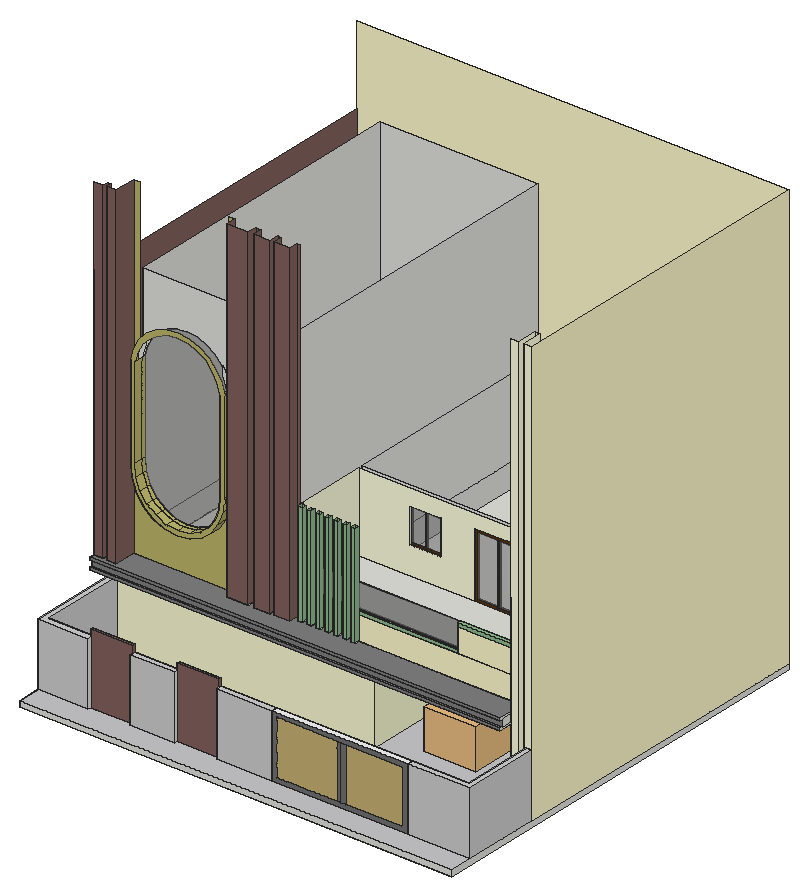
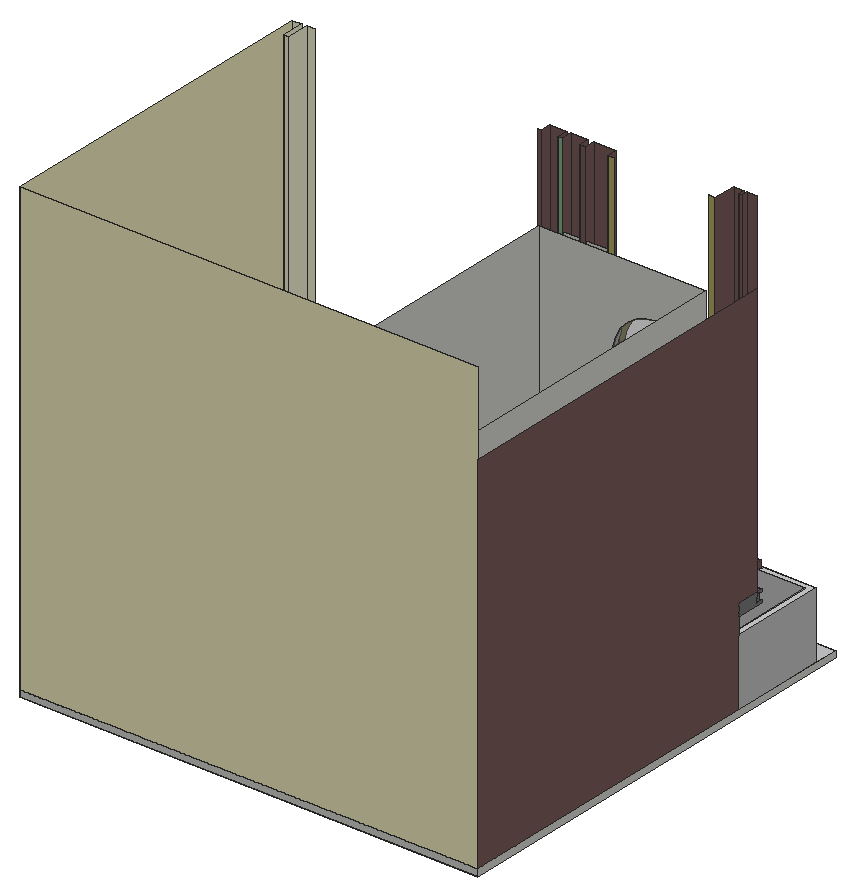
# SketchUp Ruby script. Lengths in inches.
U = 1.inch
M = Sketchup.active_model
def pt(a) = Geom::Point3d.new(a.map { |v| v * U })
def face(e, loops, mat)
  f = e.add_face(loops[0].map { |a| pt(a) })
  loops[1..].each { |l| e.add_face(l.map { |a| pt(a) }).erase! }
  f.material = f.back_material = mat if mat
  f
end
# faces: each face lists its corners as indices into pts; further lists are holes
def faces(e, pts, list, mat = nil) = list.each { |f| face(e, (f[0].is_a?(Array) ? f : [f]).map { |l| l.map { |i| pts[i] } }, mat) }
# xy, xz, yz: faces in a plane at the given z, y or x. An outline is a flat list of corners, or four numbers for a rectangle; further outlines are holes
def ring(l) = l.size == 4 ? [[l[0], l[1]], [l[2], l[1]], [l[2], l[3]], [l[0], l[3]]] : l.each_slice(2).to_a
def flat(e, list, mat, &to3) = list.each { |f| face(e, (f[0].is_a?(Array) ? f : [f]).map { |l| ring(l).map { |u, v| to3.(u, v) } }, mat) }
def xy(e, z, list, mat = nil) = flat(e, list, mat) { |x, y| [x, y, z] }
def xz(e, y, list, mat = nil) = flat(e, list, mat) { |x, z| [x, y, z] }
def yz(e, x, list, mat = nil) = flat(e, list, mat) { |y, z| [x, y, z] }
def lines(e, pts, list) = list.each { |a, b| e.add_line(pt(pts[a]), pt(pts[b])) }
# prism: a flat outline (further loops are holes) pulled along v
def prism(e, loops, v, mat = nil)
  f = face(e, loops, mat); d = Geom::Vector3d.new(v.map { |x| x * U })
  f.pushpull(f.normal.samedirection?(d) ? d.length : -d.length)
end
def box(e, o, s, mat = nil) = prism(e, [[o, [o[0] + s[0], o[1], o[2]], [o[0] + s[0], o[1] + s[1], o[2]], [o[0], o[1] + s[1], o[2]]]], [0, 0, s[2]], mat)
def at(x, y, z, deg = 0) = Geom::Transformation.translation(pt([x, y, z])) * Geom::Transformation.rotation(ORIGIN, Z_AXIS, deg.degrees)
def axes(o, x, y, z) = Geom::Transformation.new([*x, 0, *y, 0, *z, 0, *pt(o).to_a, 1])
def part(name) = M.definitions.add(name)
# library, detail: a bought-in or finely detailed component or shape, given as its bounding box
def library(name, o, s) = part(name).tap { |d| box(d.entities, o, s) }
def detail(e, o, s) = box(e.add_group.entities, o, s)
def put(e, d, t, mat = nil) = e.add_instance(d, t).tap { |i| i.material = mat if mat }
def group(e, t, mat = nil) = e.add_group.tap { |g| g.transformation = t; g.material = mat if mat }.entities
root = M.entities
M.materials.add("[0043_SaddleBrown]").color = [130, 97, 94]
M.materials.add("[0050_LemonChiffon]").color = [255, 250, 205]
M.materials.add("[0054_LightYellow]").color = [255, 255, 224]
M.materials.add("[0055_LightGoldenrodYellow]").color = [250, 250, 210]
M.materials.add("[0057_DarkKhaki]").color = [189, 183, 107]
M.materials.add("[0072_DarkSeaGreen]").color = [143, 188, 143]
M.materials.add("[0086_MediumAquamarine]").color = [102, 205, 170]
M.materials.add("[0118_Thistle]").color = [216, 191, 216]
M.materials.add("[0129_WhiteSmoke]").color = [245, 245, 245]
M.materials.add("[0133_Gray]").color = [128, 128, 128]
M.materials.add("[Cladding Siding White]").color = [207, 207, 207]
M.materials.add("[Color C08]").color = [102, 51, 0]
M.materials.add("[Color M05]").color = [114, 114, 114]
M.materials.add("[Metal Seamed]").color = [118, 119, 115]
M.materials.add("[Polished Concrete New]").color = [200, 200, 203]
M.materials.add("[Translucent Glass Gray]").color = [128, 128, 128]
M.materials["[Translucent Glass Gray]"].alpha = 0.5
M.materials.add("[Window Covering 02]").color = [199, 178, 115]
c1 = library("custom el camino",[47.5625,9.86,-8],[222.64,79.59,60.9375])
c2 = part("Group\#1")
xy(c2.entities,0,[[0,0,81.875,4.3125]],"[Color C08]")
xy(c2.entities,4.13,[[4.13,0,38.5,0.0625],[38.5,0,42.19,0.0625],[42.19,0,77.74,0.0625],[4.13,0.0625,38.5,4.3125],[38.5,0.0625,42.19,4.3125],
  [42.19,0.0625,77.74,4.3125]],"[Color C08]")
xy(c2.entities,128.34,[[4.13,0,38.5,0.0625],[42.19,0,77.74,0.0625],[4.13,0.0625,38.5,4.3125],[42.19,0.0625,77.74,4.3125]],"[Color C08]")
xy(c2.entities,132.48,[[0,0,81.875,4.3125]],"[Color C08]")
xz(c2.entities,0,[[[0,0,81.875,132.48],[4.13,4.13,4.13,128.34,38.5,128.34,38.5,4.13,42.19,4.13,42.19,128.34,77.74,128.34,77.74,4.13]]],"[Color C08]")
xz(c2.entities,0.0625,[[4.13,4.13,38.5,128.34],[42.19,4.13,77.74,128.34]],"[Translucent Glass Gray]")
xz(c2.entities,4.3125,[[[0,0,81.875,132.48],[4.13,4.13,77.74,4.13,77.74,128.34,42.19,128.34,42.19,4.13,38.5,4.13,38.5,128.34,4.13,128.34]]],"[Color C08]")
yz(c2.entities,0,[[0,0,4.3125,132.48]],"[Color C08]")
yz(c2.entities,4.13,[[0,4.13,0.0625,128.34],[0.0625,4.13,4.3125,128.34]],"[Color C08]")
yz(c2.entities,38.5,[[0,4.13,0.0625,128.34],[0.0625,4.13,4.3125,128.34]],"[Color C08]")
yz(c2.entities,42.19,[[0,4.13,0.0625,128.34],[0.0625,4.13,4.3125,128.34]],"[Color C08]")
yz(c2.entities,77.74,[[0,4.13,0.0625,128.34],[0.0625,4.13,4.3125,128.34]],"[Color C08]")
yz(c2.entities,81.875,[[0,0,4.3125,132.48]],"[Color C08]")
xy(root,0,[[0,0,657.3125,34.75],[0,34.75,657.3125,640.8125]])
xy(root,9,[[0,34.75,0,173.6875,9,173.6875,9,43.75,356.0625,43.75,356.0625,34.75,271.24,34.75,271.24,39.125,207.56,39.125,207.56,34.75,139.74,34.75,139.74,39.125,76.06,39.125,76.06,34.75],[562.44,35.125,562.44,43.75,648.3125,43.75,648.3125,152.625,657.3125,152.625,657.3125,35.125],[[624.625,152.625,624.625,631.8125,401.125,631.8125,401.125,173.6875,0,173.6875,0,640.8125,657.3125,640.8125,657.3125,152.625,644.16,152.625,644.16,183.8125,637.14,183.8125,637.14,152.625],[42.625,179.6875,395.125,631.8125]],[42.625,179.6875,395.125,631.8125]])
xy(root,9,[[0,0,657.3125,0,657.3125,35.125,562.44,35.125,562.44,34.75,271.24,34.75,271.24,39.125,207.56,39.125,207.56,34.75,139.74,34.75,139.74,39.125,76.06,39.125,76.06,34.75,0,34.75],[356.0625,34.75,562.44,43.75],[9,43.75,648.3125,43.75,648.3125,152.625,644.16,152.625,644.16,183.8125,637.14,183.8125,637.14,152.625,624.625,152.625,624.625,631.8125,401.125,631.8125,401.125,173.6875,9,173.6875]],"[Polished Concrete New]")
xy(root,105,[[356.0625,34.75,562.44,43.75]],"[0129_WhiteSmoke]")
xy(root,105,[[0,34.75,76.06,34.75,76.06,43.75,9,43.75,9,173.6875,0,173.6875],[139.74,34.75,207.56,43.75],[271.24,34.75,356.0625,43.75],[562.44,35.125,657.3125,35.125,657.3125,152.625,648.3125,152.625,648.3125,43.75,562.44,43.75]],"[Cladding Siding White]")
xy(root,115.875,[[76.06,39.125,139.74,43.75],[207.56,39.125,271.24,43.75]],"[0043_SaddleBrown]")
xy(root,123,[[42.625,179.6875,395.125,631.8125]])
xy(root,129,[[401.125,132.75,624.625,631.8125],[42.625,179.6875,395.125,631.8125]])
xy(root,129,[[0,132.75,401.125,173.6875]],"[0133_Gray]")
xy(root,132.4375,[[0,137,0,140.625,14.17,140.625,14.17,148.6875,19.125,148.6875,19.125,140.625,33.625,140.625,33.625,173.6875,187.68,173.6875,187.68,159.3125,219.81,159.3125,219.81,173.6875,228.25,173.6875,228.25,159.3125,252.93,159.3125,252.93,173.6875,289.55,173.6875,289.55,167.4375,295.8,167.4375,295.8,173.6875,302.98,173.6875,302.98,167.4375,309.23,167.4375,309.23,173.6875,316.42,173.6875,316.42,167.4375,322.67,167.4375,322.67,173.6875,329.86,173.6875,329.86,167.4375,336.11,167.4375,336.11,173.6875,343.3,173.6875,343.3,167.4375,349.55,167.4375,349.55,173.6875,356.73,173.6875,356.73,167.4375,362.98,167.4375,362.98,173.6875,370.17,173.6875,370.17,167.4375,376.42,167.4375,376.42,173.6875,624.625,173.6875,624.625,137]])
xy(root,132.4375,[[0,132.75,624.625,137]],"[0133_Gray]")
xy(root,142.6875,[[0,137,0,140.625,14.17,140.625,14.17,148.6875,19.125,148.6875,19.125,140.625,33.625,140.625,33.625,173.6875,187.68,173.6875,187.68,159.3125,219.81,159.3125,219.81,173.6875,228.25,173.6875,228.25,159.3125,252.93,159.3125,252.93,173.6875,289.55,173.6875,289.55,167.4375,295.8,167.4375,295.8,173.6875,302.98,173.6875,302.98,167.4375,309.23,167.4375,309.23,173.6875,316.42,173.6875,316.42,167.4375,322.67,167.4375,322.67,173.6875,329.86,173.6875,329.86,167.4375,336.11,167.4375,336.11,173.6875,343.3,173.6875,343.3,167.4375,349.55,167.4375,349.55,173.6875,356.73,173.6875,356.73,167.4375,362.98,167.4375,362.98,173.6875,370.17,173.6875,370.17,167.4375,376.42,167.4375,376.42,173.6875,624.625,173.6875,624.625,137]])
xy(root,142.6875,[[0,132.75,624.625,137]],"[0133_Gray]")
xy(root,146,[[0,140.625,14.17,140.625,14.17,148.6875,19.125,148.6875,19.125,140.625,33.625,140.625,33.625,173.6875,0,173.6875],[289.55,167.4375,295.8,173.6875],[302.98,167.4375,309.23,173.6875],[316.42,167.4375,322.67,173.6875],[329.86,167.4375,336.11,173.6875],
  [343.3,167.4375,349.55,173.6875],[356.73,167.4375,362.98,173.6875],[370.17,167.4375,376.42,173.6875],[42.625,179.6875,282.1875,631.8125],[287.625,291.75,624.625,631.8125]])
xy(root,146,[[0,132.75,624.625,132.75,624.625,173.6875,376.42,173.6875,376.42,167.4375,370.17,167.4375,370.17,173.6875,362.98,173.6875,362.98,167.4375,356.73,167.4375,356.73,173.6875,349.55,173.6875,349.55,167.4375,343.3,167.4375,343.3,173.6875,336.11,173.6875,336.11,167.4375,329.86,167.4375,329.86,173.6875,322.67,173.6875,322.67,167.4375,316.42,167.4375,316.42,173.6875,309.23,173.6875,309.23,167.4375,302.98,167.4375,302.98,173.6875,295.8,173.6875,295.8,167.4375,289.55,167.4375,289.55,173.6875,252.93,173.6875,252.93,159.3125,228.25,159.3125,228.25,173.6875,219.81,173.6875,219.81,159.3125,187.68,159.3125,187.68,173.6875,33.625,173.6875,33.625,140.625,19.125,140.625,19.125,148.6875,14.17,148.6875,14.17,140.625,0,140.625]],"[0133_Gray]")
xy(root,146.3125,[[258.81,159.3125,282.62,173.6875]])
xy(root,182,[[287.625,173.6875,526.86,179.6875],[526.86,173.6875,624.625,179.6875],[287.625,179.6875,624.625,179.6875,624.625,285.75,536.61,285.75,536.61,291.75,463.98,291.75,463.98,285.75,287.625,285.75]])
xy(root,187.125,[[287.625,177.42,526.86,178.24],[287.625,178.24,526.86,179.6875]])
xy(root,187.125,[[287.625,173.6875,526.86,177.42]],"[0072_DarkSeaGreen]")
xy(root,218,[[526.86,173.6875,624.625,179.6875]])
xy(root,224.1875,[[526.86,173.6875,624.625,179.6875]],"[0072_DarkSeaGreen]")
xy(root,224.1875,[[287.625,177.42,526.86,178.24]],"[Metal Seamed]")
xy(root,224.4,[[364.57,285.75,412.01,291.75]])
xy(root,224.5625,[[287.625,177.42,526.86,178.24]],"[Metal Seamed]")
xy(root,276.72,[[364.57,285.75,412.01,291.75]])
xy(root,280.8125,[[463.98,285.75,536.61,291.75]])
xz(root,0,[[0,0,657.3125,9]])
xz(root,34.75,[[0,9,76.06,105],[139.74,9,207.56,105],[271.24,9,356.0625,105]],"[Cladding Siding White]")
xz(root,34.75,[[[356.0625,9,562.44,105],[362.9,15.84,555.61,98.16]],[454.57,15.84,461.28,98.16],[461.28,15.84,467.98,98.16]],"[Color M05]")
xz(root,34.75,[[362.9,15.84,454.57,98.16],[467.98,15.84,555.61,98.16]],"[Window Covering 02]")
xz(root,35.125,[[562.44,9,657.3125,105]],"[Cladding Siding White]")
xz(root,39.125,[[76.06,9,139.74,115.875],[207.56,9,271.24,115.875]],"[0043_SaddleBrown]")
xz(root,43.75,[[76.06,105,139.74,115.875],[207.56,105,271.24,115.875]],"[0043_SaddleBrown]")
xz(root,43.75,[[356.0625,9,562.44,105]],"[0129_WhiteSmoke]")
xz(root,43.75,[[9,9,356.0625,105],[562.44,9,648.3125,105]],"[Cladding Siding White]")
xz(root,132.75,[[0,129,624.625,132.4375],[0,142.6875,624.625,146]],"[0133_Gray]")
xz(root,137,[[0,132.4375,624.625,142.6875]],"[0133_Gray]")
xz(root,140.625,[[0,132.4375,14.17,142.6875],[19.125,132.4375,33.625,142.6875],[0,142.6875,14.17,146],[19.125,142.6875,33.625,146]])
xz(root,140.625,[[0,146,14.17,655],[19.125,146,33.625,655]],"[0043_SaddleBrown]")
xz(root,148.6875,[[14.17,132.4375,19.125,142.6875],[14.17,142.6875,19.125,146]])
xz(root,148.6875,[[14.17,146,19.125,655]],"[0043_SaddleBrown]")
xz(root,152.625,[[648.3125,9,657.3125,105]])
xz(root,152.625,[[624.625,9,637.14,655],[644.16,9,648.3125,9,648.3125,105,657.3125,105,657.3125,655,644.16,655]],"[0054_LightYellow]")
xz(root,159.3125,[[187.68,132.4375,219.81,142.6875],[228.25,132.4375,252.93,142.6875],[187.68,142.6875,219.81,146],[228.25,142.6875,252.93,146]])
xz(root,159.3125,[[187.68,146,219.81,655],[228.25,146,252.93,655],[258.81,146.3125,282.62,655]],"[0043_SaddleBrown]")
xz(root,160.875,[[[111.04,201.47,130.34,204.13,148.21,211.9,163.32,224.21,174.54,240.15,181.03,258.52,182.32,277.97,182.32,417.32,177.88,433.82,169.67,448.8125,158.17,461.45,144.02,471.02,128,476.98,111.04,479.01,94.07,476.98,78.06,471.02,63.9,461.45,52.4,448.8125,44.2,433.82,39.76,417.32,39.76,277.97,41.05,258.52,47.54,240.15,58.76,224.21,73.86,211.9,91.73,204.13],[111.04,208.61,93.66,211,77.58,218,63.98,229.08,53.88,243.43,48.04,259.96,46.83,278.2,46.83,416.39,50.81,431.17,58.2,444.68,68.5625,456.0625,81.32,464.6875,95.75,470.0625,111.04,471.89,126.33,470.0625,140.75,464.6875,153.51,456.0625,163.875,444.68,171.27,431.17,175.25,416.39,175.25,278.2,174.04,259.96,168.19,243.43,158.1,229.08,144.5,218,128.41,211]]],"[0057_DarkKhaki]")
xz(root,167.4375,[[289.55,132.4375,295.8,142.6875],[302.98,132.4375,309.23,142.6875],[316.42,132.4375,322.67,142.6875],[329.86,132.4375,336.11,142.6875],[343.3,132.4375,349.55,142.6875],
  [356.73,132.4375,362.98,142.6875],[370.17,132.4375,376.42,142.6875],[289.55,142.6875,295.8,146],[302.98,142.6875,309.23,146],[316.42,142.6875,322.67,146],
  [329.86,142.6875,336.11,146],[343.3,142.6875,349.55,146],[356.73,142.6875,362.98,146],[370.17,142.6875,376.42,146]])
xz(root,167.4375,[[289.55,146,295.8,302],[302.98,146,309.23,302],[316.42,146,322.67,302],[329.86,146,336.11,302],[343.3,146,349.55,302],
  [356.73,146,362.98,302],[370.17,146,376.42,302]],"[0072_DarkSeaGreen]")
xz(root,173.6875,[[0,9,9,105],[0,129,0,146,33.625,146,33.625,132.4375,187.68,132.4375,187.68,146,219.81,146,219.81,132.4375,228.25,132.4375,228.25,146,252.93,146,252.93,132.4375,289.55,132.4375,289.55,146,295.8,146,295.8,132.4375,302.98,132.4375,302.98,146,309.23,146,309.23,132.4375,316.42,132.4375,316.42,146,322.67,146,322.67,132.4375,329.86,132.4375,329.86,146,336.11,146,336.11,132.4375,343.3,132.4375,343.3,146,349.55,146,349.55,132.4375,356.73,132.4375,356.73,146,362.98,146,362.98,132.4375,370.17,132.4375,370.17,146,376.42,146,376.42,132.4375,401.125,132.4375,401.125,129],[33.625,132.4375,187.68,142.6875],[219.81,132.4375,228.25,142.6875],[252.93,132.4375,287.625,142.6875],
  [287.625,132.4375,289.55,142.6875],[295.8,132.4375,302.98,142.6875],[309.23,132.4375,316.42,142.6875],[322.67,132.4375,329.86,142.6875],[336.11,132.4375,343.3,142.6875],
  [349.55,132.4375,356.73,142.6875],[362.98,132.4375,370.17,142.6875],[376.42,132.4375,401.125,142.6875],[401.125,132.4375,624.625,142.6875],[33.625,142.6875,187.68,146],
  [219.81,142.6875,228.25,146],[252.93,142.6875,287.625,146],[287.625,142.6875,289.55,146],[295.8,142.6875,302.98,146],[309.23,142.6875,316.42,146],
  [322.67,142.6875,329.86,146],[336.11,142.6875,343.3,146],[349.55,142.6875,356.73,146],[362.98,142.6875,370.17,146],[376.42,142.6875,401.125,146],
  [401.125,142.6875,624.625,146],[187.68,146,219.81,535],[228.25,146,252.93,535],[289.55,146,295.8,182],[302.98,146,309.23,182],
  [316.42,146,322.67,182],[329.86,146,336.11,182],[343.3,146,349.55,182],[356.73,146,362.98,182],[370.17,146,376.42,182],
  [289.55,182,295.8,187.125],[302.98,182,309.23,187.125],[316.42,182,322.67,187.125],[329.86,182,336.11,187.125],[343.3,182,349.55,187.125],
  [356.73,182,362.98,187.125],[370.17,182,376.42,187.125],[111.04,201.47,91.73,204.13,73.86,211.9,58.76,224.21,47.54,240.15,41.05,258.52,39.76,277.97,39.76,417.32,43.5,431.23,44.2,433.82,52.4,448.8125,53.1875,449.68,53.1875,435.52,50.81,431.17,46.83,416.39,46.83,278.2,48.04,259.96,53.88,243.43,63.98,229.08,77.58,218,93.66,211,111.04,208.61,128.41,211,144.5,218,158.1,229.08,168.19,243.43,174.04,259.96,175.25,278.2,175.25,416.39,171.27,431.17,169.4375,434.51,169.4375,449.07,169.67,448.8125,177.88,433.82,179.125,429.18,182.32,417.32,182.32,277.97,181.03,258.52,174.54,240.15,163.32,224.21,148.21,211.9,130.34,204.13]])
xz(root,173.6875,[[219.81,146,228.25,655],[282.62,187.125,287.625,655]],"[0043_SaddleBrown]")
xz(root,173.6875,[[376.42,146,624.625,182],[526.86,182,624.625,218]],"[0050_LemonChiffon]")
xz(root,173.6875,[[9,9,401.125,9,401.125,129,0,129,0,105,9,105]],"[0055_LightGoldenrodYellow]")
xz(root,173.6875,[[33.625,146,187.68,146,187.68,655,179.125,655,179.125,429.18,182.32,417.32,182.32,277.97,181.03,258.52,174.54,240.15,163.32,224.21,148.21,211.9,130.34,204.13,111.04,201.47,91.73,204.13,73.86,211.9,58.76,224.21,47.54,240.15,41.05,258.52,39.76,277.97,39.76,417.32,43.5,431.23,43.5,655,33.625,655]],"[0057_DarkKhaki]")
xz(root,173.6875,[[252.93,146,289.55,146,289.55,182,282.62,182,282.62,146.3125,258.81,146.3125,258.81,655,252.93,655],[295.8,146,302.98,182],[309.23,146,316.42,182],[322.67,146,329.86,182],[336.11,146,343.3,182],
  [349.55,146,356.73,182],[362.98,146,370.17,182],[282.62,182,289.55,187.125],[295.8,182,302.98,187.125],[309.23,182,316.42,187.125],
  [322.67,182,329.86,187.125],[336.11,182,343.3,187.125],[349.55,182,356.73,187.125],[362.98,182,370.17,187.125],[376.42,182,526.86,187.125],
  [289.55,187.125,295.8,302],[302.98,187.125,309.23,302],[316.42,187.125,322.67,302],[329.86,187.125,336.11,302],[343.3,187.125,349.55,302],
  [356.73,187.125,362.98,302],[370.17,187.125,376.42,302],[526.86,218,624.625,224.1875]],"[0072_DarkSeaGreen]")
xz(root,177.42,[[287.625,224.1875,526.86,224.5625]],"[Metal Seamed]")
xz(root,177.42,[[287.625,187.125,526.86,224.1875]],"[Translucent Glass Gray]")
xz(root,178.24,[[287.625,224.1875,526.86,224.5625]],"[Metal Seamed]")
xz(root,178.24,[[287.625,187.125,526.86,224.1875]],"[Translucent Glass Gray]")
xz(root,179.6875,[[42.625,9,395.125,123],[42.625,123,47.375,129],[47.375,123,52.875,129],[52.875,123,395.125,129],[42.625,129,47.375,146],
  [47.375,129,52.875,146],[52.875,129,395.125,146],[[42.625,146,282.1875,535],[111.04,208.61,128.41,211,144.5,218,158.1,229.08,168.19,243.43,174.04,259.96,175.25,278.2,175.25,416.39,171.27,431.17,163.875,444.68,153.51,456.0625,140.75,464.6875,126.33,470.0625,111.04,471.89,99.41,470.5,95.75,470.0625,81.32,464.6875,68.5625,456.0625,58.2,444.68,50.81,431.17,46.83,416.39,46.83,278.2,48.04,259.96,53.88,243.43,63.98,229.08,77.58,218,93.66,211]],[395.125,146,624.625,182],[287.625,182,395.125,187.125],
  [395.125,182,526.86,187.125],[526.86,182,624.625,218],[526.86,218,624.625,224.1875]])
xz(root,179.6875,[[111.04,208.61,93.66,211,77.58,218,63.98,229.08,53.88,243.43,48.04,259.96,46.83,278.2,46.83,416.39,50.81,431.17,58.2,444.68,68.5625,456.0625,81.32,464.6875,95.75,470.0625,99.41,470.5,111.04,471.89,126.33,470.0625,140.75,464.6875,153.51,456.0625,163.875,444.68,171.27,431.17,175.25,416.39,175.25,278.2,174.04,259.96,168.19,243.43,158.1,229.08,144.5,218,128.41,211]],"[Translucent Glass Gray]")
xz(root,183.8125,[[637.14,9,644.16,655]],"[0054_LightYellow]")
xz(root,285.75,[[[287.625,182,463.98,182,463.98,280.8125,536.61,280.8125,536.61,182,624.625,182,624.625,302,287.625,302],[364.57,224.4,412.01,276.72]]],"[0054_LightYellow]")
xz(root,291.75,[[287.625,146,624.625,182],[[287.625,182,287.625,302,624.625,302,624.625,182,536.61,182,536.61,280.8125,463.98,280.8125,463.98,182],[364.57,224.4,412.01,276.72]]])
xz(root,631.8125,[[42.625,9,395.125,123],[42.625,123,395.125,129],[42.625,129,395.125,146],[401.125,129,624.625,146],[42.625,146,282.1875,182],
  [287.625,146,624.625,182],[42.625,182,282.1875,535],[287.625,182,624.625,302]])
xz(root,631.8125,[[401.125,9,624.625,129]],"[0055_LightGoldenrodYellow]")
xz(root,640.8125,[[0,0,657.3125,9]])
xz(root,640.8125,[[0,9,657.3125,655]],"[0050_LemonChiffon]")
yz(root,0,[[0,0,640.8125,9]])
yz(root,0,[[173.6875,9,173.6875,146,140.625,146,140.625,535,640.8125,535,640.8125,9]],"[0043_SaddleBrown]")
yz(root,0,[[132.75,129,132.75,132.4375,140.625,132.4375,140.625,146,173.6875,146,173.6875,129],[137,132.4375,140.625,142.6875],[132.75,142.6875,140.625,146]],"[0133_Gray]")
yz(root,0,[[34.75,9,173.6875,105]],"[Cladding Siding White]")
yz(root,9,[[43.75,9,173.6875,105]],"[Cladding Siding White]")
yz(root,14.17,[[140.625,132.4375,148.6875,142.6875],[140.625,142.6875,148.6875,146]])
yz(root,14.17,[[140.625,146,148.6875,655]],"[0043_SaddleBrown]")
yz(root,19.125,[[140.625,132.4375,148.6875,142.6875],[140.625,142.6875,148.6875,146]])
yz(root,19.125,[[140.625,146,148.6875,655]],"[0043_SaddleBrown]")
yz(root,33.625,[[140.625,132.4375,173.6875,142.6875],[140.625,142.6875,173.6875,146]])
yz(root,33.625,[[140.625,146,173.6875,655]],"[0043_SaddleBrown]")
yz(root,39.76,[[160.875,277.97,173.6875,417.32]],"[0057_DarkKhaki]")
yz(root,42.625,[[179.6875,9,631.8125,123],[179.6875,123,631.8125,129],[179.6875,129,631.8125,146],[179.6875,146,631.8125,182],[179.6875,182,631.8125,535]])
yz(root,46.83,[[160.875,278.2,173.6875,416.39],[173.6875,278.2,179.6875,416.39]],"[0057_DarkKhaki]")
yz(root,76.06,[[34.75,9,39.125,105]])
yz(root,76.06,[[39.125,105,43.75,115.875]],"[0043_SaddleBrown]")
yz(root,139.74,[[34.75,9,39.125,105]])
yz(root,139.74,[[39.125,105,43.75,115.875]],"[0043_SaddleBrown]")
yz(root,175.25,[[160.875,278.2,173.6875,416.39],[173.6875,278.2,179.6875,416.39]],"[0057_DarkKhaki]")
yz(root,182.32,[[160.875,277.97,173.6875,417.32]],"[0057_DarkKhaki]")
yz(root,187.68,[[159.3125,132.4375,173.6875,142.6875],[159.3125,142.6875,173.6875,146]])
yz(root,187.68,[[159.3125,146,173.6875,655]],"[0043_SaddleBrown]")
yz(root,207.56,[[34.75,9,39.125,105]])
yz(root,207.56,[[39.125,105,43.75,115.875]],"[0043_SaddleBrown]")
yz(root,219.81,[[159.3125,132.4375,173.6875,142.6875],[159.3125,142.6875,173.6875,146]])
yz(root,219.81,[[159.3125,146,173.6875,655]],"[0043_SaddleBrown]")
yz(root,228.25,[[159.3125,132.4375,173.6875,142.6875],[159.3125,142.6875,173.6875,146]])
yz(root,228.25,[[159.3125,146,173.6875,655]],"[0043_SaddleBrown]")
yz(root,252.93,[[159.3125,132.4375,173.6875,142.6875],[159.3125,142.6875,173.6875,146]])
yz(root,252.93,[[159.3125,146,173.6875,655]],"[0043_SaddleBrown]")
yz(root,258.81,[[159.3125,146.3125,173.6875,655]],"[0043_SaddleBrown]")
yz(root,271.24,[[34.75,9,39.125,105]])
yz(root,271.24,[[39.125,105,43.75,115.875]],"[0043_SaddleBrown]")
yz(root,282.1875,[[179.6875,146,631.8125,182],[179.6875,182,631.8125,535]])
yz(root,282.62,[[159.3125,146.3125,173.6875,655]],"[0043_SaddleBrown]")
yz(root,287.625,[[291.75,146,631.8125,182],[291.75,182,631.8125,302],[173.6875,187.125,177.42,187.125,177.42,224.5625,178.24,224.5625,178.24,187.125,179.6875,187.125,179.6875,302,173.6875,302],[177.42,187.125,178.24,224.1875]])
yz(root,287.625,[[179.6875,182,285.75,302]],"[0054_LightYellow]")
yz(root,287.625,[[177.42,224.1875,178.24,224.5625]],"[Metal Seamed]")
yz(root,289.55,[[167.4375,132.4375,173.6875,142.6875],[167.4375,142.6875,173.6875,146]])
yz(root,289.55,[[167.4375,146,173.6875,302]],"[0072_DarkSeaGreen]")
yz(root,295.8,[[167.4375,132.4375,173.6875,142.6875],[167.4375,142.6875,173.6875,146]])
yz(root,295.8,[[167.4375,146,173.6875,302]],"[0072_DarkSeaGreen]")
yz(root,302.98,[[167.4375,132.4375,173.6875,142.6875],[167.4375,142.6875,173.6875,146]])
yz(root,302.98,[[167.4375,146,173.6875,302]],"[0072_DarkSeaGreen]")
yz(root,309.23,[[167.4375,132.4375,173.6875,142.6875],[167.4375,142.6875,173.6875,146]])
yz(root,309.23,[[167.4375,146,173.6875,302]],"[0072_DarkSeaGreen]")
yz(root,316.42,[[167.4375,132.4375,173.6875,142.6875],[167.4375,142.6875,173.6875,146]])
yz(root,316.42,[[167.4375,146,173.6875,302]],"[0072_DarkSeaGreen]")
yz(root,322.67,[[167.4375,132.4375,173.6875,142.6875],[167.4375,142.6875,173.6875,146]])
yz(root,322.67,[[167.4375,146,173.6875,302]],"[0072_DarkSeaGreen]")
yz(root,329.86,[[167.4375,132.4375,173.6875,142.6875],[167.4375,142.6875,173.6875,146]])
yz(root,329.86,[[167.4375,146,173.6875,302]],"[0072_DarkSeaGreen]")
yz(root,336.11,[[167.4375,132.4375,173.6875,142.6875],[167.4375,142.6875,173.6875,146]])
yz(root,336.11,[[167.4375,146,173.6875,302]],"[0072_DarkSeaGreen]")
yz(root,343.3,[[167.4375,132.4375,173.6875,142.6875],[167.4375,142.6875,173.6875,146]])
yz(root,343.3,[[167.4375,146,173.6875,302]],"[0072_DarkSeaGreen]")
yz(root,349.55,[[167.4375,132.4375,173.6875,142.6875],[167.4375,142.6875,173.6875,146]])
yz(root,349.55,[[167.4375,146,173.6875,302]],"[0072_DarkSeaGreen]")
yz(root,356.0625,[[34.75,9,43.75,105]],"[0129_WhiteSmoke]")
yz(root,356.73,[[167.4375,132.4375,173.6875,142.6875],[167.4375,142.6875,173.6875,146]])
yz(root,356.73,[[167.4375,146,173.6875,302]],"[0072_DarkSeaGreen]")
yz(root,362.98,[[167.4375,132.4375,173.6875,142.6875],[167.4375,142.6875,173.6875,146]])
yz(root,362.98,[[167.4375,146,173.6875,302]],"[0072_DarkSeaGreen]")
yz(root,364.57,[[285.75,224.4,291.75,276.72]])
yz(root,370.17,[[167.4375,132.4375,173.6875,142.6875],[167.4375,142.6875,173.6875,146]])
yz(root,370.17,[[167.4375,146,173.6875,302]],"[0072_DarkSeaGreen]")
yz(root,376.42,[[167.4375,132.4375,173.6875,142.6875],[167.4375,142.6875,173.6875,146]])
yz(root,376.42,[[167.4375,146,173.6875,302]],"[0072_DarkSeaGreen]")
yz(root,395.125,[[179.6875,9,631.8125,123],[179.6875,123,631.8125,129]])
yz(root,401.125,[[173.6875,9,631.8125,129]],"[0055_LightGoldenrodYellow]")
yz(root,412.01,[[285.75,224.4,291.75,276.72]])
yz(root,463.98,[[285.75,182,291.75,280.8125]])
yz(root,526.86,[[173.6875,182,179.6875,187.125],[177.42,187.125,178.24,218],[178.24,187.125,179.6875,218],[177.42,218,178.24,224.1875],[178.24,218,179.6875,224.1875]])
yz(root,526.86,[[173.6875,187.125,177.42,218],[173.6875,218,177.42,224.1875]],"[0072_DarkSeaGreen]")
yz(root,526.86,[[177.42,224.1875,178.24,224.5625]],"[Metal Seamed]")
yz(root,536.61,[[285.75,182,291.75,280.8125]])
yz(root,562.44,[[35.125,9,43.75,105]],"[Cladding Siding White]")
yz(root,624.625,[[132.75,129,152.625,132.4375],[137,132.4375,152.625,142.6875],[152.625,132.4375,173.6875,142.6875],[132.75,142.6875,152.625,146],[152.625,142.6875,173.6875,146],
  [173.6875,146,179.6875,182],[179.6875,146,291.75,182],[291.75,146,631.8125,182],[173.6875,182,179.6875,218],[179.6875,182,285.75,302],
  [285.75,182,291.75,302],[291.75,182,631.8125,302],[173.6875,218,179.6875,224.1875]])
yz(root,624.625,[[152.625,146,152.625,302,179.6875,302,179.6875,224.1875,173.6875,224.1875,173.6875,146]],"[0054_LightYellow]")
yz(root,624.625,[[152.625,9,631.8125,129]],"[0118_Thistle]")
yz(root,637.14,[[152.625,9,183.8125,655]],"[0054_LightYellow]")
yz(root,644.16,[[152.625,9,183.8125,655]],"[0054_LightYellow]")
yz(root,648.3125,[[43.75,9,152.625,105]],"[Cladding Siding White]")
yz(root,657.3125,[[0,0,640.8125,9]])
yz(root,657.3125,[[152.625,9,640.8125,655]],"[0050_LemonChiffon]")
yz(root,657.3125,[[35.125,9,152.625,105]],"[Cladding Siding White]")
p = [[91.73,173.6875,204.13],[111.04,173.6875,201.47],[111.04,160.875,201.47],[91.73,160.875,204.13],[130.34,173.6875,204.13],[130.34,160.875,204.13],
  [73.86,173.6875,211.9],[73.86,160.875,211.9],[148.21,173.6875,211.9],[148.21,160.875,211.9],[111.04,173.6875,208.61],[93.66,173.6875,211],
  [93.66,160.875,211],[111.04,160.875,208.61],[128.41,173.6875,211],[128.41,160.875,211],[111.04,179.6875,208.61],[93.66,179.6875,211],
  [128.41,179.6875,211],[77.58,173.6875,218],[77.58,160.875,218],[144.5,173.6875,218],[144.5,160.875,218],[77.58,179.6875,218],
  [144.5,179.6875,218],[58.76,173.6875,224.21],[58.76,160.875,224.21],[163.32,173.6875,224.21],[163.32,160.875,224.21],[63.98,173.6875,229.08],
  [63.98,160.875,229.08],[158.1,173.6875,229.08],[158.1,160.875,229.08],[63.98,179.6875,229.08],[158.1,179.6875,229.08],[47.54,173.6875,240.15],
  [47.54,160.875,240.15],[174.54,173.6875,240.15],[174.54,160.875,240.15],[53.88,173.6875,243.43],[53.88,160.875,243.43],[168.19,173.6875,243.43],
  [168.19,160.875,243.43],[53.88,179.6875,243.43],[168.19,179.6875,243.43],[41.05,173.6875,258.52],[41.05,160.875,258.52],[181.03,173.6875,258.52],
  [181.03,160.875,258.52],[48.04,173.6875,259.96],[48.04,160.875,259.96],[174.04,173.6875,259.96],[174.04,160.875,259.96],[48.04,179.6875,259.96],
  [174.04,179.6875,259.96],[39.76,173.6875,277.97],[39.76,160.875,277.97],[182.32,173.6875,277.97],[182.32,160.875,277.97],[46.83,173.6875,278.2],
  [46.83,160.875,278.2],[175.25,173.6875,278.2],[175.25,160.875,278.2],[46.83,179.6875,278.2],[175.25,179.6875,278.2],[287.625,179.6875,146],
  [287.625,173.6875,146],[287.625,179.6875,182]]
faces(root,p,[[0,1,2,3],[1,4,5,2],[6,0,3,7],[4,8,9,5],[10,11,12,13],[14,10,13,15],[11,10,16,17],[10,14,18,16],
  [11,19,20,12],[21,14,15,22],[19,11,17,23],[14,21,24,18],[25,6,7,26],[8,27,28,9],[19,29,30,20],[31,21,22,32],
  [29,19,23,33],[21,31,34,24],[35,25,26,36],[27,37,38,28],[29,39,40,30],[41,31,32,42],[39,29,33,43],[31,41,44,34],
  [45,35,36,46],[37,47,48,38],[39,49,50,40],[51,41,42,52],[49,39,43,53],[41,51,54,44],[55,45,46,56],[47,57,58,48],
  [49,59,60,50],[61,51,52,62],[59,49,53,63],[51,61,64,54]],"[0057_DarkKhaki]")
lines(root,p,[[65,66],[65,67]])
put(root,c1,at(540.65,155.875,17,90))
put(root,c2,axes([463.98,285.75,182],[0.88702,0,0],[0,0.5,0],[0,0,0.74589]),"[0086_MediumAquamarine]")
put(root,c2,axes([364.34,287.8125,224.4],[0.58222,0,0],[0,0.38115,0],[0,0,0.39488]))
